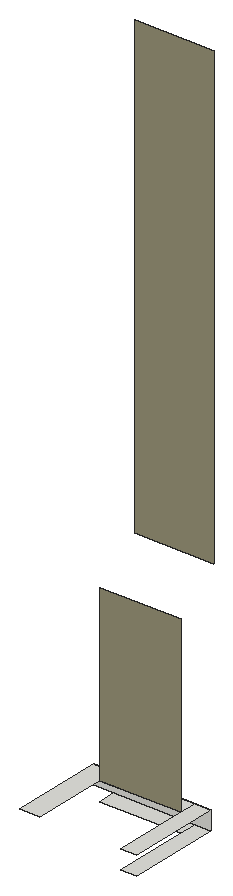
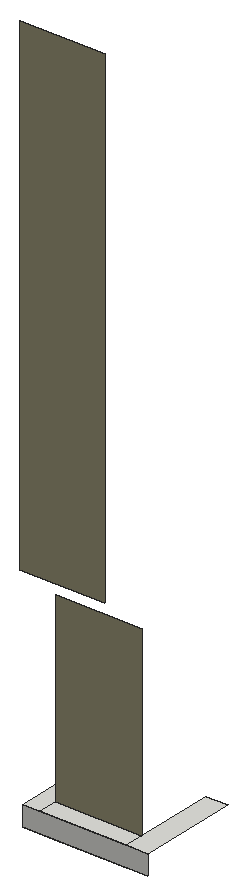
# SketchUp Ruby script. Lengths in inches.
U = 1.inch
M = Sketchup.active_model
def pt(a) = Geom::Point3d.new(a.map { |v| v * U })
def face(e, loops, mat)
  f = e.add_face(loops[0].map { |a| pt(a) })
  loops[1..].each { |l| e.add_face(l.map { |a| pt(a) }).erase! }
  f.material = f.back_material = mat if mat
  f
end
# faces: each face lists its corners as indices into pts; further lists are holes
def faces(e, pts, list, mat = nil) = list.each { |f| face(e, (f[0].is_a?(Array) ? f : [f]).map { |l| l.map { |i| pts[i] } }, mat) }
# xy, xz, yz: faces in a plane at the given z, y or x. An outline is a flat list of corners, or four numbers for a rectangle; further outlines are holes
def ring(l) = l.size == 4 ? [[l[0], l[1]], [l[2], l[1]], [l[2], l[3]], [l[0], l[3]]] : l.each_slice(2).to_a
def flat(e, list, mat, &to3) = list.each { |f| face(e, (f[0].is_a?(Array) ? f : [f]).map { |l| ring(l).map { |u, v| to3.(u, v) } }, mat) }
def xy(e, z, list, mat = nil) = flat(e, list, mat) { |x, y| [x, y, z] }
def xz(e, y, list, mat = nil) = flat(e, list, mat) { |x, z| [x, y, z] }
def yz(e, x, list, mat = nil) = flat(e, list, mat) { |y, z| [x, y, z] }
def lines(e, pts, list) = list.each { |a, b| e.add_line(pt(pts[a]), pt(pts[b])) }
# prism: a flat outline (further loops are holes) pulled along v
def prism(e, loops, v, mat = nil)
  f = face(e, loops, mat); d = Geom::Vector3d.new(v.map { |x| x * U })
  f.pushpull(f.normal.samedirection?(d) ? d.length : -d.length)
end
def box(e, o, s, mat = nil) = prism(e, [[o, [o[0] + s[0], o[1], o[2]], [o[0] + s[0], o[1] + s[1], o[2]], [o[0], o[1] + s[1], o[2]]]], [0, 0, s[2]], mat)
def at(x, y, z, deg = 0) = Geom::Transformation.translation(pt([x, y, z])) * Geom::Transformation.rotation(ORIGIN, Z_AXIS, deg.degrees)
def axes(o, x, y, z) = Geom::Transformation.new([*x, 0, *y, 0, *z, 0, *pt(o).to_a, 1])
def part(name) = M.definitions.add(name)
# library, detail: a bought-in or finely detailed component or shape, given as its bounding box
def library(name, o, s) = part(name).tap { |d| box(d.entities, o, s) }
def detail(e, o, s) = box(e.add_group.entities, o, s)
def put(e, d, t, mat = nil) = e.add_instance(d, t).tap { |i| i.material = mat if mat }
def group(e, t, mat = nil) = e.add_group.tap { |g| g.transformation = t; g.material = mat if mat }.entities
root = M.entities
M.materials.add("[Stone Coursed Rough]").color = [155, 150, 122]
xy(root,92.87,[[297.85,203.17,301.1,221.48],[281.86,217.98,297.85,221.48]])
xy(root,96.63,[[277.93,203.17,281.86,221.48],[297.85,203.17,301.1,221.48],[281.86,217.98,297.85,221.48]])
xz(root,217.98,[[281.86,96.63,297.85,130.875]],"[Stone Coursed Rough]")
xz(root,221.48,[[277.93,92.87,301.1,96.63]])
xz(root,225.17,[[283.04,137.875,298.6,228.8125]],"[Stone Coursed Rough]")
